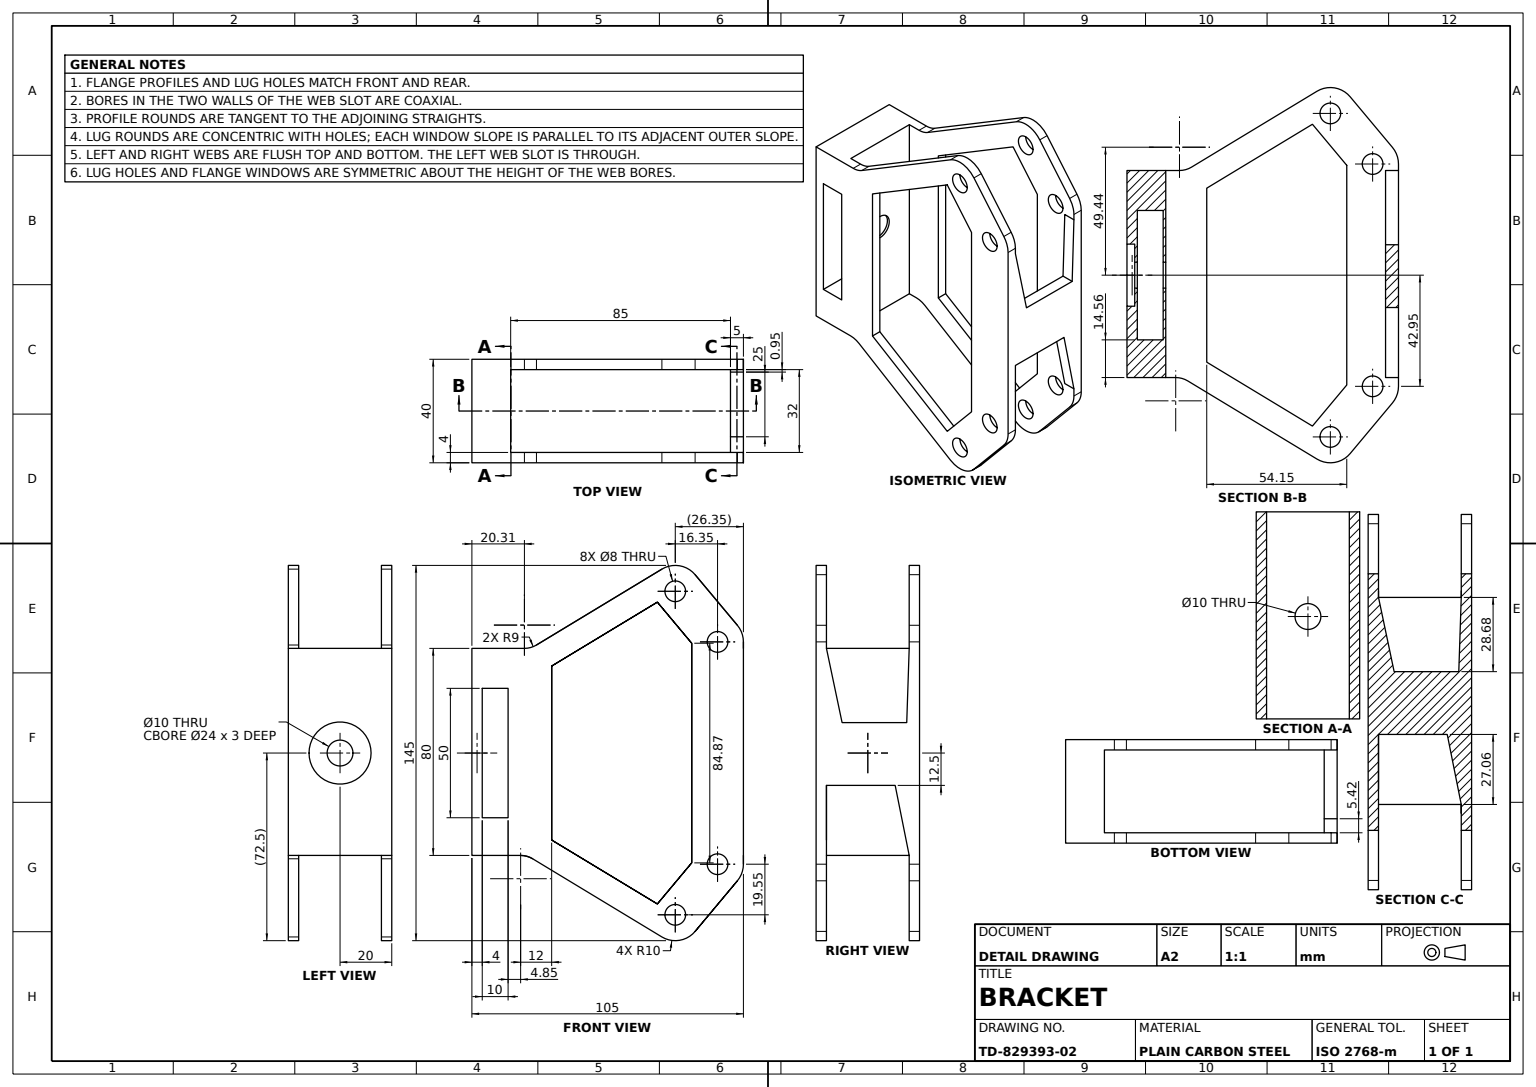
solid
v1 (7.146632,25,20)
v2 (7.146632,25,-20)
e1 v1 v2 LINE
v3 (-2.853368,25,20)
e2 v1 v3 LINE
v4 (-2.853368,25,-20)
e3 v3 v4 LINE
e4 v2 v4 LINE
face PLANE(AX(P(7.146632,25,20),D(0,-1,0),D(1,0,0))) [-e1 e2 e3 -e4]
v5 (84.146632,42.95,20)
v6 (84.146632,42.95,16)
e5 v5 v6 LINE
v7 (92.146632,42.95,16)
e6 v7 v6 CIRCLE(AX(P(88.146632,42.95,16),D(0,0,1),D(1,0,0)),4)
v8 (92.146632,42.95,20)
e7 v8 v7 LINE
e8 v8 v5 CIRCLE(AX(P(88.146632,42.95,20),D(0,0,1),D(1,0,0)),4)
face CYL(AX(P(88.146632,42.95,20),D(0,0,-1),D(-1,0,0)),4) rev [e5 -e6 -e7 e8]
v9 (98.146632,40.441447,16)
v10 (93.146632,40.441447,16)
e9 v9 v10 LINE
v11 (98.146632,11.757126,9.950879)
e10 v9 v11 LINE
v12 (93.146632,11.757126,9.950879)
e11 v12 v11 LINE
e12 v10 v12 LINE
face PLANE(AX(P(58.146632,40.441447,16),D(0,-0.206347439,0.978478786),D(0,-0.978478786,-0.206347439))) rev [-e9 e10 -e11 -e12]
v13 (92.146632,42.95,-16)
v14 (84.146632,42.95,-16)
e13 v13 v14 CIRCLE(AX(P(88.146632,42.95,-16),D(0,0,-1),D(-1,0,0)),4)
v15 (92.146632,42.95,-20)
e14 v13 v15 LINE
v16 (84.146632,42.95,-20)
e15 v16 v15 CIRCLE(AX(P(88.146632,42.95,-20),D(0,0,1),D(1,0,0)),4)
e16 v14 v16 LINE
face CYL(AX(P(88.146632,42.95,20),D(0,0,-1),D(-1,0,0)),4) rev [-e13 e14 -e15 -e16]
v17 (75.796632,-62.5,-16)
v18 (75.796632,-62.5,-20)
e17 v17 v18 LINE
v19 (67.796632,-62.5,-16)
e18 v19 v17 CIRCLE(AX(P(71.796632,-62.5,-16),D(0,0,-1),D(-1,0,0)),4)
v20 (67.796632,-62.5,-20)
e19 v19 v20 LINE
e20 v18 v20 CIRCLE(AX(P(71.796632,-62.5,-20),D(0,0,1),D(-1,0,0)),4)
face CYL(AX(P(71.796632,-62.5,20),D(0,0,-1),D(-1,0,0)),4) rev [-e17 -e18 e19 -e20]
v21 (93.146632,-12.5,-10.579626)
v22 (98.146632,-12.5,-10.579626)
e21 v21 v22 LINE
v23 (98.146632,-12.5,16)
e22 v22 v23 LINE
v24 (93.146632,-12.5,16)
e23 v24 v23 LINE
e24 v21 v24 LINE
face PLANE(AX(P(58.146632,-12.5,16),D(0,1,0),D(0,0,1))) rev [e21 e22 -e23 -e24]
v25 (98.146632,40.441447,-16)
v26 (93.146632,40.441447,-16)
e25 v25 v26 LINE
v27 (93.146632,11.757126,-15.049121)
e26 v27 v26 LINE
v28 (98.146632,11.757126,-15.049121)
e27 v27 v28 LINE
e28 v28 v25 LINE
face PLANE(AX(P(58.146632,40.441447,-16),D(0,-0.033131594,-0.999450998),D(0,0.999450998,-0.033131594))) rev [e25 -e26 e27 e28]
v29 (-2.853368,-25,20)
v30 (-2.853368,-25,-20)
e29 v29 v30 LINE
v31 (7.146632,-25,20)
e30 v29 v31 LINE
v32 (7.146632,-25,-20)
e31 v31 v32 LINE
e32 v30 v32 LINE
face PLANE(AX(P(7.146632,-25,20),D(0,1,0),D(0,0,1))) [-e29 e30 e31 -e32]
v33 (16.651884,-40.856045,-20)
v34 (66.624129,-71.058342,-20)
e33 v33 v34 LINE
v35 (66.624129,-71.058342,-16)
e34 v35 v34 LINE
v36 (16.651884,-40.856045,-16)
e35 v35 v36 LINE
e36 v36 v33 LINE
face PLANE(AX(P(16.651884,-40.856045,20),D(0.517250282,0.855834181,0),D(-0.855834181,0.517250282,0))) rev [e33 -e34 e35 e36]
v37 (-3.853368,0,-12)
v38 (-6.853368,0,-12)
e37 v37 v38 LINE
v39 (-6.853368,0,12)
e38 v38 v39 CIRCLE(AX(P(-6.853368,0,0),D(-1,0,0),D(0,0,1)),12)
v40 (-3.853368,0,12)
e39 v40 v39 LINE
e40 v37 v40 CIRCLE(AX(P(-3.853368,0,0),D(-1,0,0),D(0,0,1)),12)
face CYL(AX(P(-3.853368,0,0),D(-1,0,0),D(0,0,1)),12) rev [e37 e38 -e39 -e40]
v41 (23.996632,-33.610568,20)
v42 (64.86918,-58.313177,20)
e41 v41 v42 LINE
v43 (64.86918,-58.313177,16)
e42 v42 v43 LINE
v44 (23.996632,-33.610568,16)
e43 v44 v43 LINE
e44 v41 v44 LINE
face PLANE(AX(P(64.86918,-58.313177,20),D(0.517250282,0.855834181,0),D(-0.855834181,0.517250282,0))) [e41 e42 -e43 -e44]
e45 v24 v10 LINE
e46 v12 v27 LINE
v45 (93.146632,-39.558553,-16)
e47 v45 v26 LINE
e48 v45 v21 LINE
face PLANE(AX(P(93.146632,-72.5,16),D(1,0,0),D(0,0,-1))) rev [e24 e45 e12 e46 e26 -e47 e48]
v46 (78.146632,-42.43708,20)
e49 v42 v46 LINE
v47 (78.146632,-42.43708,16)
e50 v46 v47 LINE
e51 v43 v47 LINE
face PLANE(AX(P(78.146632,-42.43708,20),D(-0.767094424,0.641534211,0),D(-0.641534211,-0.767094424,0))) [-e42 e49 e50 -e51]
v48 (75.796632,62.5,-20)
v49 (67.796632,62.5,-20)
e52 v48 v49 CIRCLE(AX(P(71.796632,62.5,-20),D(0,0,1),D(1,0,0)),4)
v50 (75.796632,62.5,-16)
e53 v50 v48 LINE
v51 (67.796632,62.5,-16)
e54 v51 v50 CIRCLE(AX(P(71.796632,62.5,-16),D(0,0,-1),D(-1,0,0)),4)
e55 v51 v49 LINE
face CYL(AX(P(71.796632,62.5,20),D(0,0,-1),D(-1,0,0)),4) rev [-e52 -e53 -e54 e55]
v52 (98.146632,-39.558553,-16)
e56 v52 v45 LINE
e57 v52 v22 LINE
face PLANE(AX(P(58.146632,-39.558553,-16),D(0,0.196417985,-0.980520257),D(0,0.980520257,0.196417985))) rev [-e48 -e56 e57 -e21]
e58 v11 v28 LINE
face PLANE(AX(P(58.146632,11.757126,9.950879),D(0,-1,0),D(0,0,-1))) rev [-e46 e11 e58 -e27]
v53 (-2.853368,0,5)
v54 (-2.853368,0,-5)
e59 v53 v54 CIRCLE(AX(P(-2.853368,0,0),D(1,0,0),D(0,0,-1)),5)
v55 (-3.853368,0,-5)
e60 v54 v55 LINE
v56 (-3.853368,0,5)
e61 v56 v55 CIRCLE(AX(P(-3.853368,0,0),D(1,0,0),D(0,0,1)),5)
e62 v53 v56 LINE
face CYL(AX(P(33.146632,0,0),D(-1,0,0),D(0,0,1)),5) rev [e59 e60 -e61 -e62]
v57 (11.996632,-39.558553,-16)
e63 v36 v57 CIRCLE(AX(P(11.996632,-48.558553,-16),D(0,0,1),D(-1,0,0)),9)
v58 (11.996632,-39.558553,-20)
e64 v57 v58 LINE
e65 v58 v33 CIRCLE(AX(P(11.996632,-48.558553,-20),D(0,0,-1),D(-1,0,0)),9)
face CYL(AX(P(11.996632,-48.558553,20),D(0,0,-1),D(-1,0,0)),9) rev [-e36 e63 e64 e65]
v59 (64.86918,58.313177,-16)
v60 (78.146632,42.43708,-16)
e66 v59 v60 LINE
v61 (64.86918,58.313177,-20)
e67 v59 v61 LINE
v62 (78.146632,42.43708,-20)
e68 v62 v61 LINE
e69 v60 v62 LINE
face PLANE(AX(P(78.146632,42.43708,20),D(-0.767094424,-0.641534211,0),D(0.641534211,-0.767094424,0))) [-e66 e67 -e68 -e69]
v63 (11.996632,-39.558553,16)
v64 (16.651884,-40.856045,16)
e70 v63 v64 CIRCLE(AX(P(11.996632,-48.558553,16),D(0,0,-1),D(1,0,0)),9)
v65 (16.651884,-40.856045,20)
e71 v65 v64 LINE
v66 (11.996632,-39.558553,20)
e72 v66 v65 CIRCLE(AX(P(11.996632,-48.558553,20),D(0,0,-1),D(-1,0,0)),9)
e73 v66 v63 LINE
face CYL(AX(P(11.996632,-48.558553,20),D(0,0,-1),D(-1,0,0)),9) rev [e70 -e71 -e72 e73]
v67 (13.457454,40.441447,-16)
v68 (13.457454,40.441447,-20)
e74 v67 v68 LINE
v69 (-6.853368,40.441447,-20)
e75 v68 v69 LINE
v70 (-6.853368,40.441447,20)
e76 v70 v69 LINE
v71 (13.457454,40.441447,20)
e77 v71 v70 LINE
v72 (13.457454,40.441447,16)
e78 v71 v72 LINE
v73 (8.146632,40.441447,16)
e79 v72 v73 LINE
v74 (8.146632,40.441447,-16)
e80 v73 v74 LINE
e81 v74 v67 LINE
face PLANE(AX(P(13.457454,40.441447,20),D(0,-1,0),D(0,0,-1))) rev [e74 e75 -e76 -e77 e78 e79 e80 e81]
v75 (23.996632,33.610568,-16)
v76 (23.996632,33.610568,-20)
e82 v75 v76 LINE
e83 v61 v76 LINE
e84 v75 v59 LINE
face PLANE(AX(P(64.86918,58.313177,20),D(0.517250282,-0.855834181,0),D(0.855834181,0.517250282,0))) [e82 -e83 -e67 -e84]
v77 (23.996632,33.610568,16)
e85 v77 v44 LINE
v78 (23.996632,33.610568,20)
e86 v78 v77 LINE
e87 v78 v41 LINE
face PLANE(AX(P(23.996632,33.610568,20),D(1,0,0),D(0,0,-1))) [-e85 -e86 e87 e44]
v79 (7.146632,0,-5)
v80 (7.146632,0,5)
e88 v79 v80 CIRCLE(AX(P(7.146632,0,0),D(-1,0,0),D(0,0,1)),5)
v81 (8.146632,0,5)
e89 v81 v80 LINE
v82 (8.146632,0,-5)
e90 v82 v81 CIRCLE(AX(P(8.146632,0,0),D(-1,0,0),D(0,0,1)),5)
e91 v82 v79 LINE
face CYL(AX(P(33.146632,0,0),D(-1,0,0),D(0,0,1)),5) rev [e88 -e89 -e90 e91]
e92 v17 v19 CIRCLE(AX(P(71.796632,-62.5,-16),D(0,0,-1),D(-1,0,0)),4)
e93 v20 v18 CIRCLE(AX(P(71.796632,-62.5,-20),D(0,0,1),D(-1,0,0)),4)
face CYL(AX(P(71.796632,-62.5,20),D(0,0,-1),D(-1,0,0)),4) rev [-e92 e17 -e93 -e19]
v83 (79.467576,-68.915342,20)
v84 (79.467576,-68.915342,16)
e94 v83 v84 LINE
v85 (95.817576,-49.365342,16)
e95 v84 v85 LINE
v86 (95.817576,-49.365342,20)
e96 v86 v85 LINE
e97 v83 v86 LINE
face PLANE(AX(P(79.467576,-68.915342,20),D(-0.767094424,0.641534211,0),D(-0.641534211,-0.767094424,0))) rev [e94 e95 -e96 -e97]
v87 (18.112707,41.738939,20)
v88 (18.112707,41.738939,16)
e98 v87 v88 LINE
e99 v88 v72 CIRCLE(AX(P(13.457454,49.441447,16),D(0,0,-1),D(1,0,0)),9)
e100 v87 v71 CIRCLE(AX(P(13.457454,49.441447,20),D(0,0,-1),D(-1,0,0)),9)
face CYL(AX(P(13.457454,49.441447,20),D(0,0,-1),D(-1,0,0)),9) rev [e98 e99 -e78 -e100]
v89 (78.146632,-42.43708,-16)
v90 (78.146632,-42.43708,-20)
e101 v89 v90 LINE
v91 (64.86918,-58.313177,-20)
e102 v91 v90 LINE
v92 (64.86918,-58.313177,-16)
e103 v92 v91 LINE
e104 v89 v92 LINE
face PLANE(AX(P(78.146632,-42.43708,20),D(-0.767094424,0.641534211,0),D(-0.641534211,-0.767094424,0))) [e101 -e102 -e103 -e104]
e105 v49 v48 CIRCLE(AX(P(71.796632,62.5,-20),D(0,0,1),D(1,0,0)),4)
v93 (84.146632,-42.95,-20)
v94 (92.146632,-42.95,-20)
e106 v93 v94 CIRCLE(AX(P(88.146632,-42.95,-20),D(0,0,1),D(-1,0,0)),4)
e107 v94 v93 CIRCLE(AX(P(88.146632,-42.95,-20),D(0,0,1),D(-1,0,0)),4)
e108 v15 v16 CIRCLE(AX(P(88.146632,42.95,-20),D(0,0,1),D(1,0,0)),4)
e109 v32 v2 LINE
e110 v4 v30 LINE
v95 (-6.853368,-39.558553,-20)
e111 v95 v58 LINE
e112 v69 v95 LINE
v96 (18.112707,41.738939,-20)
e113 v96 v68 CIRCLE(AX(P(13.457454,49.441447,-20),D(0,0,-1),D(-1,0,0)),9)
v97 (66.624129,71.058342,-20)
e114 v97 v96 LINE
v98 (79.467576,68.915342,-20)
e115 v98 v97 CIRCLE(AX(P(71.796632,62.5,-20),D(0,0,1),D(-1,0,0)),10)
v99 (95.817576,49.365342,-20)
e116 v99 v98 LINE
v100 (98.146632,42.95,-20)
e117 v100 v99 CIRCLE(AX(P(88.146632,42.95,-20),D(0,0,1),D(-1,0,0)),10)
v101 (98.146632,-42.95,-20)
e118 v101 v100 LINE
v102 (95.817576,-49.365342,-20)
e119 v102 v101 CIRCLE(AX(P(88.146632,-42.95,-20),D(0,0,1),D(1,0,0)),10)
v103 (79.467576,-68.915342,-20)
e120 v103 v102 LINE
e121 v34 v103 CIRCLE(AX(P(71.796632,-62.5,-20),D(0,0,1),D(1,0,0)),10)
v104 (23.996632,-33.610568,-20)
e122 v76 v104 LINE
e123 v104 v91 LINE
e124 v90 v62 LINE
face PLANE(AX(P(13.457454,49.441447,-20),D(0,0,-1),D(-1,0,0))) [e105 e52] [e106 e107] [e108 e15] [e32 e109 e4 e110] [-e65 -e111 -e112 -e75 -e113 -e114 -e115 -e116 -e117 -e118 -e119 -e120 -e121 -e33] [e83 e122 e123 e102 e124 e68] [e93 e20]
v105 (75.796632,62.5,20)
v106 (75.796632,62.5,16)
e125 v105 v106 LINE
v107 (67.796632,62.5,16)
e126 v107 v106 CIRCLE(AX(P(71.796632,62.5,16),D(0,0,1),D(1,0,0)),4)
v108 (67.796632,62.5,20)
e127 v108 v107 LINE
e128 v108 v105 CIRCLE(AX(P(71.796632,62.5,20),D(0,0,1),D(1,0,0)),4)
face CYL(AX(P(71.796632,62.5,20),D(0,0,-1),D(-1,0,0)),4) rev [e125 -e126 -e127 e128]
v109 (64.86918,58.313177,20)
e129 v109 v78 LINE
v110 (64.86918,58.313177,16)
e130 v110 v77 LINE
e131 v109 v110 LINE
face PLANE(AX(P(64.86918,58.313177,20),D(0.517250282,-0.855834181,0),D(0.855834181,0.517250282,0))) [e129 e86 -e130 -e131]
v111 (98.146632,42.95,20)
v112 (95.817576,49.365342,20)
e132 v111 v112 CIRCLE(AX(P(88.146632,42.95,20),D(0,0,1),D(-1,0,0)),10)
v113 (98.146632,42.95,16)
e133 v111 v113 LINE
v114 (95.817576,49.365342,16)
e134 v113 v114 CIRCLE(AX(P(88.146632,42.95,16),D(0,0,1),D(1,0,0)),10)
e135 v112 v114 LINE
face CYL(AX(P(88.146632,42.95,20),D(0,0,-1),D(-1,0,0)),10) [-e132 e133 e134 -e135]
e136 v55 v56 CIRCLE(AX(P(-3.853368,0,0),D(1,0,0),D(0,0,1)),5)
e137 v40 v37 CIRCLE(AX(P(-3.853368,0,0),D(-1,0,0),D(0,0,1)),12)
face PLANE(AX(P(-3.853368,0,0),D(-1,0,0),D(0,0,1))) [e61 e136] [e137 e40]
v115 (75.796632,-62.5,20)
v116 (67.796632,-62.5,20)
e138 v115 v116 CIRCLE(AX(P(71.796632,-62.5,20),D(0,0,1),D(-1,0,0)),4)
v117 (67.796632,-62.5,16)
e139 v116 v117 LINE
v118 (75.796632,-62.5,16)
e140 v118 v117 CIRCLE(AX(P(71.796632,-62.5,16),D(0,0,1),D(1,0,0)),4)
e141 v115 v118 LINE
face CYL(AX(P(71.796632,-62.5,20),D(0,0,-1),D(-1,0,0)),4) rev [e138 e139 -e140 -e141]
v119 (95.817576,-49.365342,-16)
e142 v119 v102 LINE
v120 (79.467576,-68.915342,-16)
e143 v119 v120 LINE
e144 v120 v103 LINE
face PLANE(AX(P(79.467576,-68.915342,20),D(-0.767094424,0.641534211,0),D(-0.641534211,-0.767094424,0))) rev [-e142 e143 e144 e120]
e145 v81 v82 CIRCLE(AX(P(8.146632,0,0),D(-1,0,0),D(0,0,1)),5)
v121 (8.146632,-39.558553,16)
e146 v121 v73 LINE
v122 (8.146632,-39.558553,-16)
e147 v122 v121 LINE
e148 v122 v74 LINE
face PLANE(AX(P(8.146632,-72.5,16),D(-1,0,0),D(0,0,1))) rev [e90 e145] [-e146 -e147 e148 -e80]
v123 (79.467576,68.915342,16)
v124 (66.624129,71.058342,16)
e149 v123 v124 CIRCLE(AX(P(71.796632,62.5,16),D(0,0,1),D(1,0,0)),10)
v125 (66.624129,71.058342,20)
e150 v125 v124 LINE
v126 (79.467576,68.915342,20)
e151 v126 v125 CIRCLE(AX(P(71.796632,62.5,20),D(0,0,1),D(-1,0,0)),10)
e152 v126 v123 LINE
face CYL(AX(P(71.796632,62.5,20),D(0,0,-1),D(-1,0,0)),10) [e149 -e150 -e151 e152]
v127 (-6.853368,-39.558553,20)
e153 v127 v95 LINE
e154 v57 v122 LINE
e155 v121 v63 LINE
e156 v127 v66 LINE
face PLANE(AX(P(11.996632,-39.558553,20),D(0,1,0),D(-1,0,0))) rev [e153 e111 -e64 e154 e147 e155 -e73 -e156]
e157 v54 v53 CIRCLE(AX(P(-2.853368,0,0),D(1,0,0),D(0,0,-1)),5)
e158 v3 v29 LINE
face PLANE(AX(P(-2.853368,-25,20),D(1,0,0),D(0,0,-1))) [-e59 -e157] [-e110 -e3 e158 e29]
v128 (98.146632,-42.95,-16)
e159 v128 v101 LINE
e160 v128 v119 CIRCLE(AX(P(88.146632,-42.95,-16),D(0,0,-1),D(-1,0,0)),10)
face CYL(AX(P(88.146632,-42.95,20),D(0,0,-1),D(-1,0,0)),10) [e119 -e159 e160 e142]
v129 (84.146632,-42.95,-16)
v130 (92.146632,-42.95,-16)
e161 v129 v130 CIRCLE(AX(P(88.146632,-42.95,-16),D(0,0,-1),D(-1,0,0)),4)
e162 v130 v129 CIRCLE(AX(P(88.146632,-42.95,-16),D(0,0,-1),D(-1,0,0)),4)
e163 v60 v89 LINE
v131 (23.996632,-33.610568,-16)
e164 v92 v131 LINE
e165 v131 v75 LINE
e166 v50 v51 CIRCLE(AX(P(71.796632,62.5,-16),D(0,0,-1),D(-1,0,0)),4)
v132 (18.112707,41.738939,-16)
v133 (66.624129,71.058342,-16)
e167 v132 v133 LINE
e168 v67 v132 CIRCLE(AX(P(13.457454,49.441447,-16),D(0,0,1),D(-1,0,0)),9)
e169 v120 v35 CIRCLE(AX(P(71.796632,-62.5,-16),D(0,0,-1),D(-1,0,0)),10)
e170 v52 v128 LINE
v134 (98.146632,42.95,-16)
e171 v134 v25 LINE
v135 (95.817576,49.365342,-16)
e172 v135 v134 CIRCLE(AX(P(88.146632,42.95,-16),D(0,0,-1),D(0,1,0)),10)
v136 (79.467576,68.915342,-16)
e173 v136 v135 LINE
e174 v133 v136 CIRCLE(AX(P(71.796632,62.5,-16),D(0,0,-1),D(-1,0,0)),10)
e175 v14 v13 CIRCLE(AX(P(88.146632,42.95,-16),D(0,0,-1),D(-1,0,0)),4)
face PLANE(AX(P(93.146632,-72.5,-16),D(0,0,-1),D(-1,0,0))) rev [e161 e162] [e66 e163 e104 e164 e165 e84] [e54 e166] [e18 e92] [-e167 -e168 -e81 -e148 -e154 -e63 -e35 -e169 -e143 -e160 -e170 e56 e47 -e25 -e171 -e172 -e173 -e174] [e175 e13]
e176 v70 v127 LINE
e177 v39 v38 CIRCLE(AX(P(-6.853368,0,0),D(-1,0,0),D(0,0,1)),12)
face PLANE(AX(P(-6.853368,-39.558553,20),D(1,0,0),D(0,0,-1))) rev [-e153 -e176 e76 e112] [-e38 -e177]
e178 v130 v94 LINE
e179 v129 v93 LINE
face CYL(AX(P(88.146632,-42.95,20),D(0,0,-1),D(-1,0,0)),4) rev [-e107 -e178 -e161 e179]
v137 (78.146632,42.43708,20)
v138 (78.146632,42.43708,16)
e180 v137 v138 LINE
e181 v47 v138 LINE
e182 v46 v137 LINE
face PLANE(AX(P(78.146632,-42.43708,20),D(-1,0,0),D(0,0,1))) [e180 -e181 -e50 e182]
v139 (92.146632,-42.95,20)
v140 (84.146632,-42.95,20)
e183 v139 v140 CIRCLE(AX(P(88.146632,-42.95,20),D(0,0,1),D(-1,0,0)),4)
v141 (84.146632,-42.95,16)
e184 v140 v141 LINE
v142 (92.146632,-42.95,16)
e185 v142 v141 CIRCLE(AX(P(88.146632,-42.95,16),D(0,0,1),D(1,0,0)),4)
e186 v139 v142 LINE
face CYL(AX(P(88.146632,-42.95,20),D(0,0,-1),D(-1,0,0)),4) rev [e183 e184 -e185 -e186]
e187 v141 v142 CIRCLE(AX(P(88.146632,-42.95,16),D(0,0,1),D(1,0,0)),4)
e188 v140 v139 CIRCLE(AX(P(88.146632,-42.95,20),D(0,0,1),D(-1,0,0)),4)
face CYL(AX(P(88.146632,-42.95,20),D(0,0,-1),D(-1,0,0)),4) rev [-e187 -e184 e188 e186]
face PLANE(AX(P(78.146632,-42.43708,20),D(-1,0,0),D(0,0,1))) [e69 -e124 -e101 -e163]
face CYL(AX(P(71.796632,62.5,20),D(0,0,-1),D(-1,0,0)),4) rev [-e105 -e55 -e166 e53]
face CYL(AX(P(-3.853368,0,0),D(-1,0,0),D(0,0,1)),12) rev [-e137 e39 e177 -e37]
e189 v136 v98 LINE
e190 v135 v99 LINE
face PLANE(AX(P(79.467576,68.915342,20),D(-0.767094424,-0.641534211,0),D(0.641534211,-0.767094424,0))) rev [-e189 e173 e190 e116]
e191 v131 v104 LINE
face PLANE(AX(P(64.86918,-58.313177,20),D(0.517250282,0.855834181,0),D(-0.855834181,0.517250282,0))) [-e164 e103 -e123 -e191]
e192 v124 v88 LINE
e193 v125 v87 LINE
face PLANE(AX(P(18.112707,41.738939,20),D(0.517250282,-0.855834181,0),D(0.855834181,0.517250282,0))) rev [e192 -e98 -e193 e150]
e194 v106 v107 CIRCLE(AX(P(71.796632,62.5,16),D(0,0,1),D(1,0,0)),4)
e195 v105 v108 CIRCLE(AX(P(71.796632,62.5,20),D(0,0,1),D(1,0,0)),4)
face CYL(AX(P(71.796632,62.5,20),D(0,0,-1),D(-1,0,0)),4) rev [e127 -e194 -e125 e195]
e196 v80 v79 CIRCLE(AX(P(7.146632,0,0),D(-1,0,0),D(0,0,1)),5)
face CYL(AX(P(33.146632,0,0),D(-1,0,0),D(0,0,1)),5) rev [e89 e196 -e91 -e145]
e197 v137 v109 LINE
e198 v138 v110 LINE
face PLANE(AX(P(78.146632,42.43708,20),D(-0.767094424,-0.641534211,0),D(0.641534211,-0.767094424,0))) [e197 e131 -e198 -e180]
e199 v5 v8 CIRCLE(AX(P(88.146632,42.95,20),D(0,0,1),D(1,0,0)),4)
e200 v112 v126 LINE
v143 (66.624129,-71.058342,20)
e201 v65 v143 LINE
e202 v143 v83 CIRCLE(AX(P(71.796632,-62.5,20),D(0,0,1),D(1,0,0)),10)
v144 (98.146632,-42.95,20)
e203 v86 v144 CIRCLE(AX(P(88.146632,-42.95,20),D(0,0,1),D(1,0,0)),10)
e204 v144 v111 LINE
e205 v31 v1 LINE
e206 v116 v115 CIRCLE(AX(P(71.796632,-62.5,20),D(0,0,1),D(-1,0,0)),4)
face PLANE(AX(P(13.457454,49.441447,20),D(0,0,-1),D(-1,0,0))) rev [-e199 -e8] [e132 e200 e151 e193 e100 e77 e176 e156 e72 e201 e202 e97 e203 e204] [-e183 -e188] [-e129 -e197 -e182 -e49 -e41 -e87] [-e128 -e195] [-e158 -e2 -e205 -e30] [-e206 -e138]
face CYL(AX(P(33.146632,0,0),D(-1,0,0),D(0,0,1)),5) rev [-e136 -e60 e157 e62]
e207 v133 v97 LINE
face CYL(AX(P(71.796632,62.5,20),D(0,0,-1),D(-1,0,0)),10) [-e207 e174 e189 e115]
face CYL(AX(P(88.146632,42.95,20),D(0,0,-1),D(-1,0,0)),4) rev [-e14 -e175 e16 -e108]
face CYL(AX(P(88.146632,-42.95,20),D(0,0,-1),D(-1,0,0)),4) rev [e178 -e106 -e179 -e162]
e208 v6 v7 CIRCLE(AX(P(88.146632,42.95,16),D(0,0,1),D(1,0,0)),4)
face CYL(AX(P(88.146632,42.95,20),D(0,0,-1),D(-1,0,0)),4) rev [e7 -e208 -e5 e199]
v145 (66.624129,-71.058342,16)
e209 v64 v145 LINE
e210 v143 v145 LINE
face PLANE(AX(P(16.651884,-40.856045,20),D(0.517250282,0.855834181,0),D(-0.855834181,0.517250282,0))) rev [e209 -e210 -e201 e71]
face PLANE(AX(P(7.146632,-25,20),D(-1,0,0),D(0,0,1))) [-e196 -e88] [e1 -e109 -e31 e205]
e211 v145 v84 CIRCLE(AX(P(71.796632,-62.5,16),D(0,0,1),D(1,0,0)),10)
face CYL(AX(P(71.796632,-62.5,20),D(0,0,-1),D(-1,0,0)),10) [e210 e211 -e94 -e202]
e212 v114 v123 LINE
face PLANE(AX(P(79.467576,68.915342,20),D(-0.767094424,-0.641534211,0),D(0.641534211,-0.767094424,0))) rev [e212 -e152 -e200 e135]
e213 v132 v96 LINE
face CYL(AX(P(13.457454,49.441447,20),D(0,0,-1),D(-1,0,0)),9) rev [e113 -e74 e168 e213]
face CYL(AX(P(71.796632,-62.5,20),D(0,0,-1),D(-1,0,0)),10) [e34 e121 -e144 e169]
e214 v9 v113 LINE
v146 (98.146632,-42.95,16)
e215 v144 v146 LINE
e216 v146 v23 LINE
e217 v134 v100 LINE
face PLANE(AX(P(98.146632,42.95,20),D(-1,0,0),D(0,0,1))) rev [-e58 -e10 e214 -e133 -e204 e215 e216 -e22 -e57 e170 e159 e118 -e217 e171 -e28]
e218 v117 v118 CIRCLE(AX(P(71.796632,-62.5,16),D(0,0,1),D(1,0,0)),4)
face CYL(AX(P(71.796632,-62.5,20),D(0,0,-1),D(-1,0,0)),4) rev [e141 -e218 -e139 e206]
e219 v85 v146 CIRCLE(AX(P(88.146632,-42.95,16),D(0,0,1),D(1,0,0)),10)
face CYL(AX(P(88.146632,-42.95,20),D(0,0,-1),D(-1,0,0)),10) [-e203 e96 e219 -e215]
face CYL(AX(P(88.146632,42.95,20),D(0,0,-1),D(-1,0,0)),10) [e117 -e190 e172 e217]
face PLANE(AX(P(93.146632,-72.5,16),D(0,0,1),D(1,0,0))) rev [e198 e130 e85 e43 e51 e181] [e187 e185] [e23 -e216 -e219 -e95 -e211 -e209 -e70 -e155 e146 -e79 -e99 -e192 -e149 -e212 -e134 -e214 e9 -e45] [e140 e218] [e6 e208] [e126 e194]
face PLANE(AX(P(23.996632,33.610568,20),D(1,0,0),D(0,0,-1))) [e191 -e122 -e82 -e165]
face PLANE(AX(P(18.112707,41.738939,20),D(0.517250282,-0.855834181,0),D(0.855834181,0.517250282,0))) rev [e167 e207 e114 -e213]
